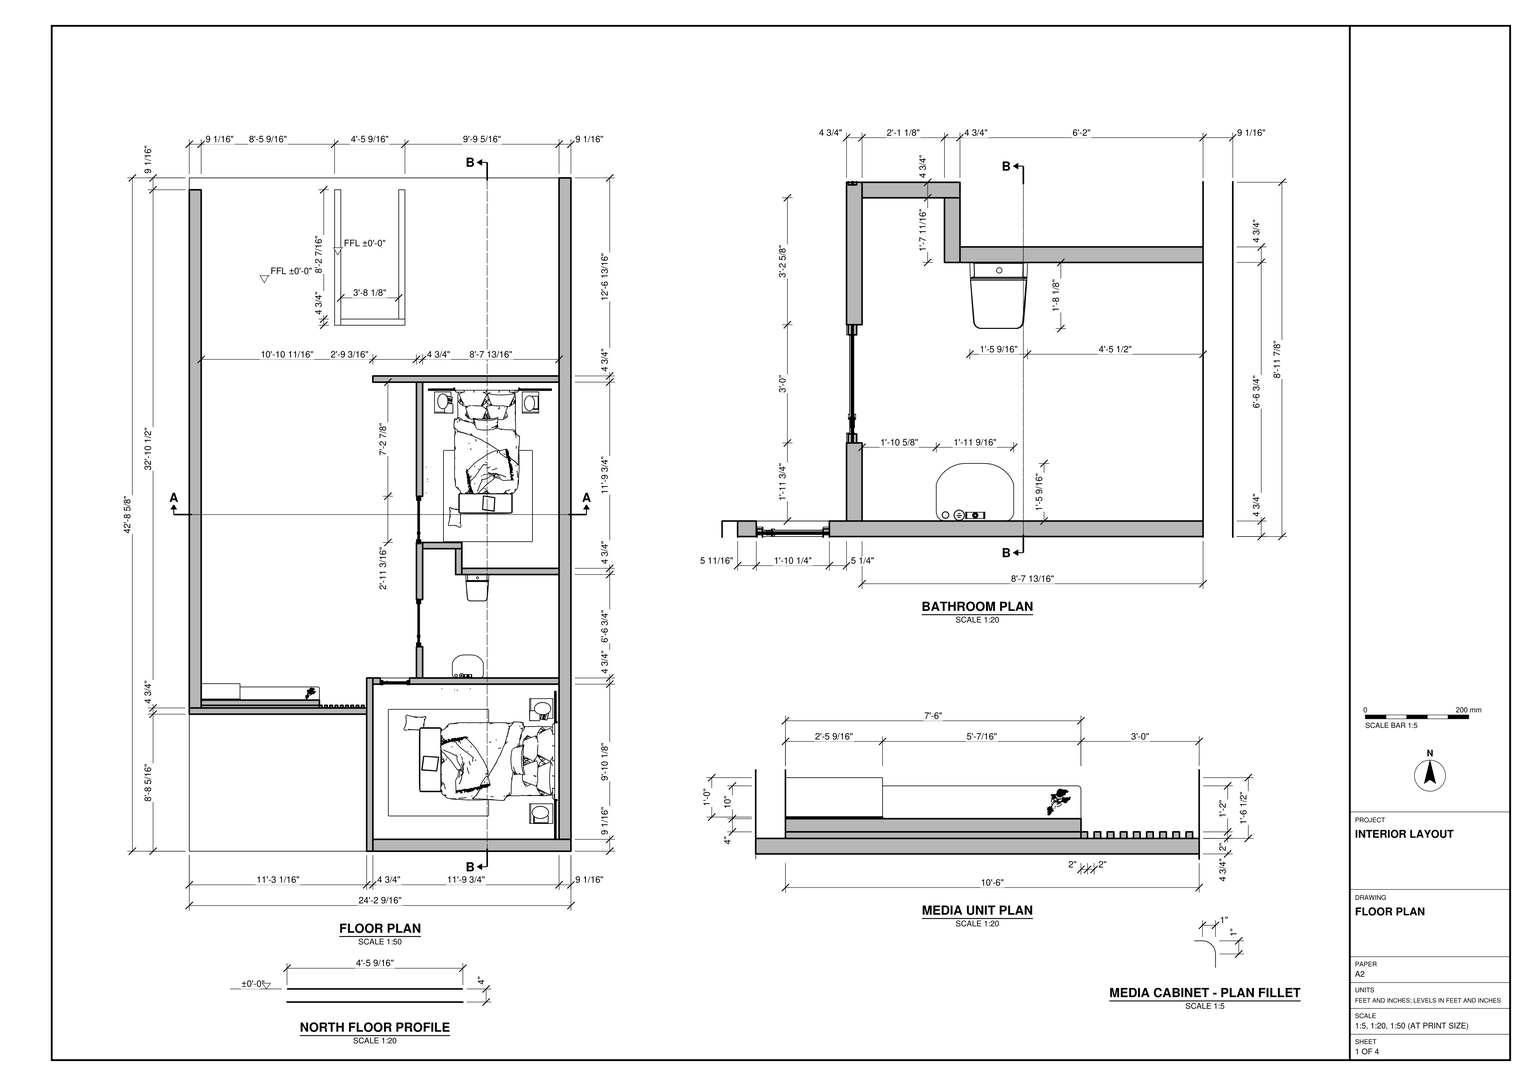
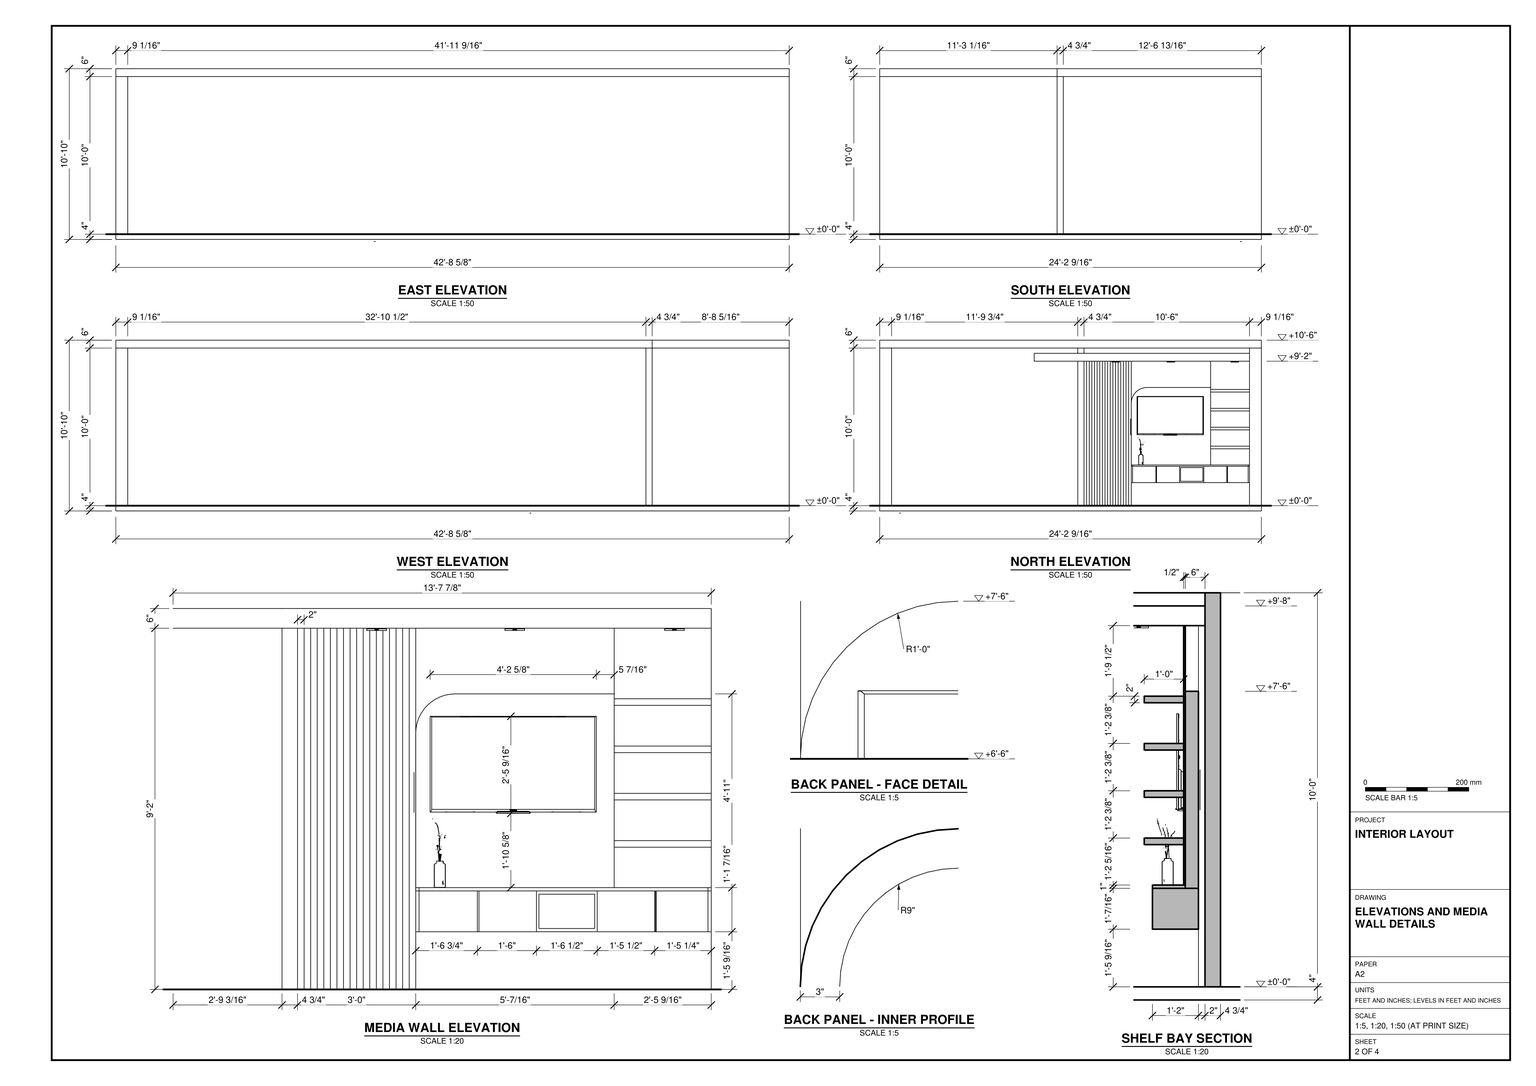
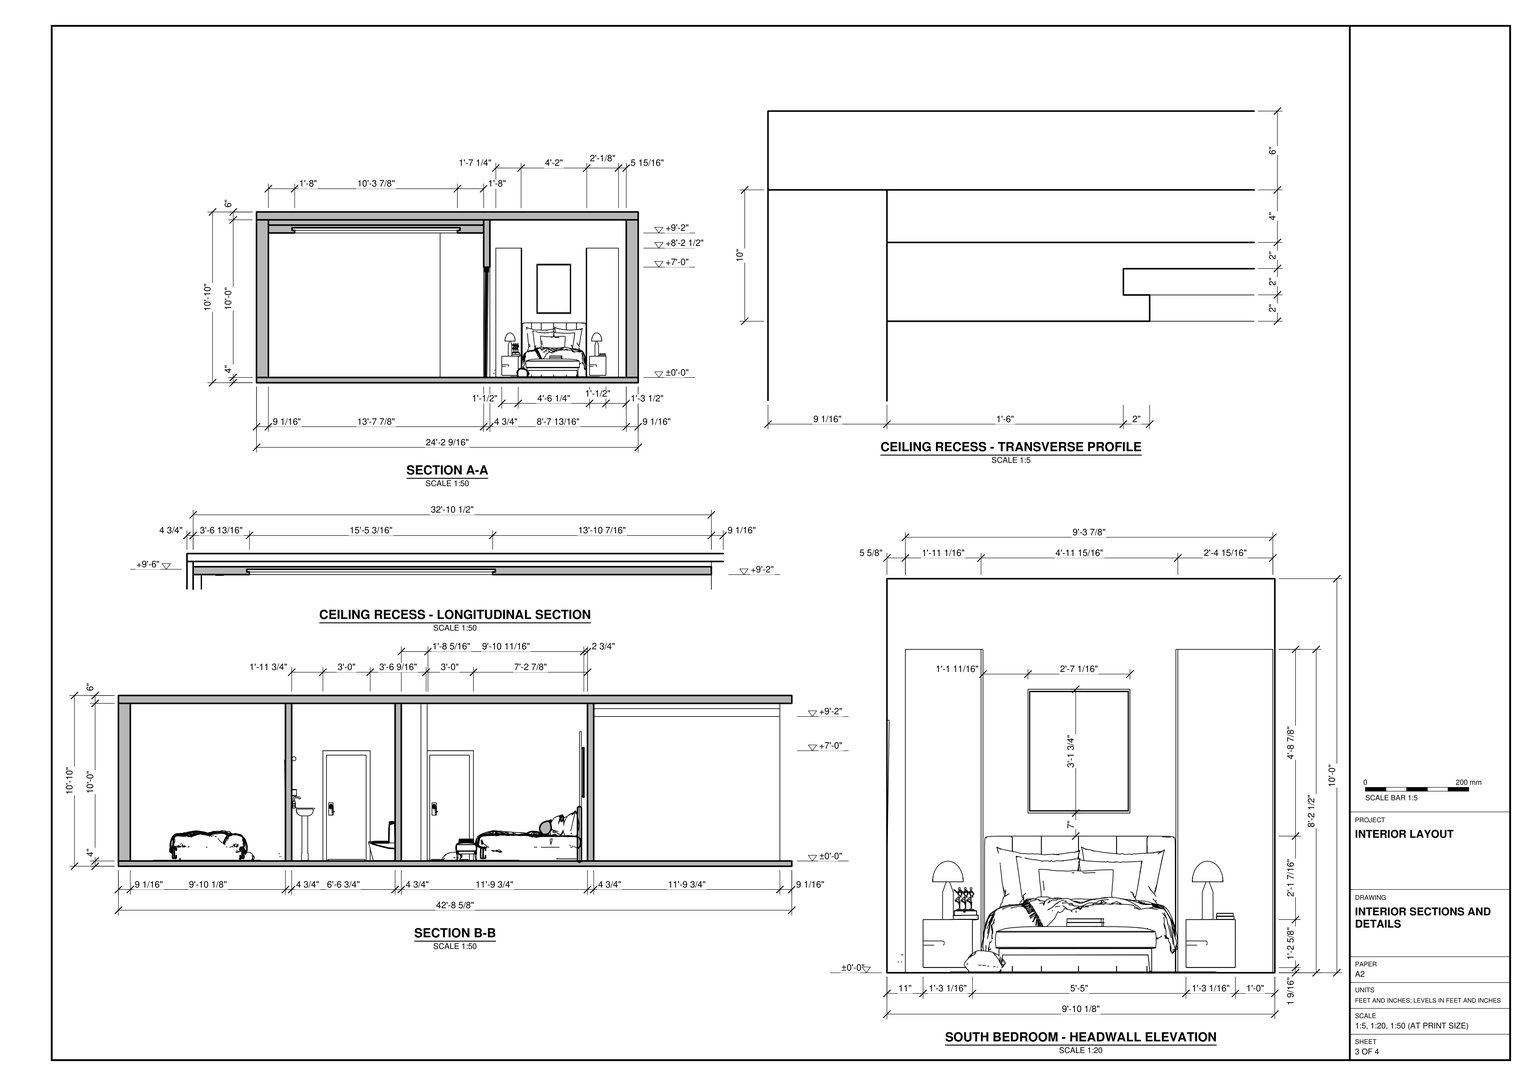
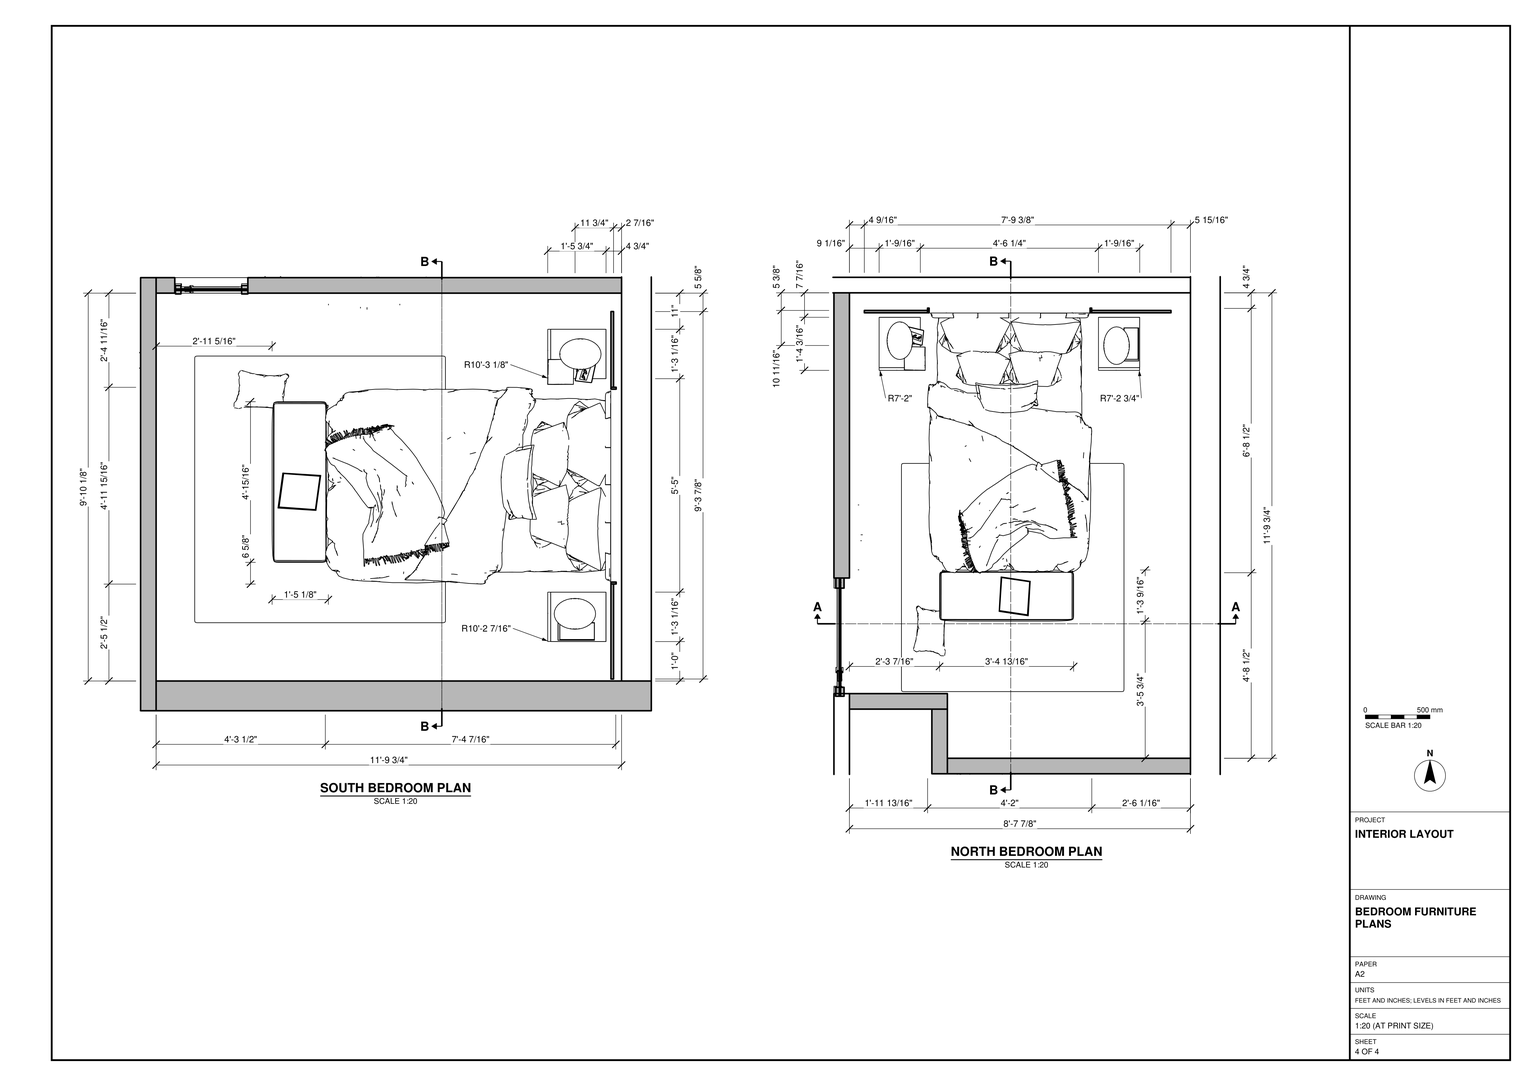
Build the furnished interior in SketchUp from task_files/diagram_01.pdf. Work in feet and inches. Set the finished floor at ±0'-0". The overall model is 24'-2 9/16" wide, 42'-8 5/8" long and 10'-10" high, including the floor and roof slabs.

Use the floor plan to set out the open area on the west and the two bedrooms on the east, with the bathroom between them. Follow the drawn wall thicknesses, partition returns and door openings, including the stepped wall behind the toilet. Match the north floor profile to the detail. Use the sections to establish the clear room height and to shape the stepped ceiling recess above the open area.

Place each bed and its bedside units in the orientation shown. Use the south bedroom elevation to size and position the headwall panels around the bed. Build the media wall from its plan, elevation and shelf section: distinguish the vertical slats, rounded screen back panel, suspended low cabinet and open shelf bay. Decor and loose items may be any suitable library components.

Keep the walls, slabs and roof as separate groups or components, and group each furniture or joinery piece separately. Use components for repeated parts. Save one SketchUp model as output_files/two_bedroom_interior_with_media_wall.skp.

# SketchUp Ruby script. Lengths in inches.
U = 1.inch
M = Sketchup.active_model
def pt(a) = Geom::Point3d.new(a.map { |v| v * U })
def face(e, loops, mat)
  f = e.add_face(loops[0].map { |a| pt(a) })
  loops[1..].each { |l| e.add_face(l.map { |a| pt(a) }).erase! }
  f.material = f.back_material = mat if mat
  f
end
# faces: each face lists its corners as indices into pts; further lists are holes
def faces(e, pts, list, mat = nil) = list.each { |f| face(e, (f[0].is_a?(Array) ? f : [f]).map { |l| l.map { |i| pts[i] } }, mat) }
# xy, xz, yz: faces in a plane at the given z, y or x. An outline is a flat list of corners, or four numbers for a rectangle; further outlines are holes
def ring(l) = l.size == 4 ? [[l[0], l[1]], [l[2], l[1]], [l[2], l[3]], [l[0], l[3]]] : l.each_slice(2).to_a
def flat(e, list, mat, &to3) = list.each { |f| face(e, (f[0].is_a?(Array) ? f : [f]).map { |l| ring(l).map { |u, v| to3.(u, v) } }, mat) }
def xy(e, z, list, mat = nil) = flat(e, list, mat) { |x, y| [x, y, z] }
def xz(e, y, list, mat = nil) = flat(e, list, mat) { |x, z| [x, y, z] }
def yz(e, x, list, mat = nil) = flat(e, list, mat) { |y, z| [x, y, z] }
def lines(e, pts, list) = list.each { |a, b| e.add_line(pt(pts[a]), pt(pts[b])) }
# prism: a flat outline (further loops are holes) pulled along v
def prism(e, loops, v, mat = nil)
  f = face(e, loops, mat); d = Geom::Vector3d.new(v.map { |x| x * U })
  f.pushpull(f.normal.samedirection?(d) ? d.length : -d.length)
end
def box(e, o, s, mat = nil) = prism(e, [[o, [o[0] + s[0], o[1], o[2]], [o[0] + s[0], o[1] + s[1], o[2]], [o[0], o[1] + s[1], o[2]]]], [0, 0, s[2]], mat)
def at(x, y, z, deg = 0) = Geom::Transformation.translation(pt([x, y, z])) * Geom::Transformation.rotation(ORIGIN, Z_AXIS, deg.degrees)
def axes(o, x, y, z) = Geom::Transformation.new([*x, 0, *y, 0, *z, 0, *pt(o).to_a, 1])
def part(name) = M.definitions.add(name)
# library, detail: a bought-in or finely detailed component or shape, given as its bounding box
def library(name, o, s) = part(name).tap { |d| box(d.entities, o, s) }
def detail(e, o, s) = box(e.add_group.entities, o, s)
def put(e, d, t, mat = nil) = e.add_instance(d, t).tap { |i| i.material = mat if mat }
def group(e, t, mat = nil) = e.add_group.tap { |g| g.transformation = t; g.material = mat if mat }.entities
root = M.entities
M.materials.add("0176 AP 7460 CRYSTAL RIVER").color = [209, 232, 226]
M.materials.add("0196 AP 8700 DIVINITY").color = [235, 221, 218]
M.materials.add("[Carrera Marble]").color = [207, 207, 207]
c1 = library("feets plan.dwg",[0,0,0],[290.55,512.6,0.01])
c2 = library("Nhatay-Combo+Bed-Modern+stylist+(35) (1)",[-205.01,128.15,-1.01],[153.05,130.41,99.44])
c3 = library("porta+4 (2)",[0.2,-5.42,1.33],[46.55,4.72,83.21])
c4 = library("3x5 small bath",[0,-13.07,0],[75.24,78.74,85])
c5 = part("Square post")
xy(c5.entities,0,[[0,0,2,2]])
xy(c5.entities,110,[[0,0,2,2]])
xz(c5.entities,0,[[0,0,2,110]])
xz(c5.entities,2,[[0,0,2,110]],"0176 AP 7460 CRYSTAL RIVER")
yz(c5.entities,0,[[0,0,2,110]],"0176 AP 7460 CRYSTAL RIVER")
yz(c5.entities,2,[[0,0,2,110]],"0176 AP 7460 CRYSTAL RIVER")
c6 = part("Shelf panel")
box(c6.entities,[0,0,0],[29.5625,12,2])
c7 = part("Group260\#1")
p = [[0,0,0],[0,0,-5.07],[-2.27,0,-5.07],[14.78,-1.625,0],[-14.78,-1.625,0],[14.78,1.625,0],
  [14.78,0,0],[-14.78,1.625,0],[2.27,0,-5.07],[-14.78,0,0],[0,0,-8.2]]
lines(c7.entities,p,[[0,1],[1,2],[3,4],[5,6],[7,5],[1,8],[9,0],[0,6],[8,10],[4,9],[6,3],[2,10],
  [9,7]])
c8 = part("Rectangle Light")
put(c8.entities,c7,at(0,0,0))
c9 = library("Flat panel television",[0,5.31,3.09],[110.25,6.46,64.42])
c10 = library("Sphere Light",[-21.15,-21.15,-21.15],[42.3,42.3,42.3])
c11 = library("Group\#21",[-0.5,-0.5,0],[91,4.5,60])
c12 = library("Group\#23",[-0.5,-0.5,-0.1],[128.88,190.2,0.2])
c13 = library("Group\#64",[-6.9375,-9.94,6.79],[29.29,38.38,46.85])
c14 = library("Group\#49",[0,0,0],[6,6,0.5])
put(root,c1,at(0,0,0))
put(root,c2,axes([23.37,-29.09,0.05],[0,-0.74598,0],[1,0,0],[0,0,1]))
put(root,c3,axes([145.56,131.89,0.12],[0.47368,0,0],[0,1,0],[0,0,0.90881]))
put(root,c4,at(275.5,197.5625,-5.625,-180))
put(root,c3,axes([171.1,155.51,-1.38],[0,0.77339,0],[-1,0,0],[0,0,1.01001]))
put(root,c3,axes([171.1,234.09,-1.38],[0,0.77339,0],[-1,0,0],[0,0,1.01001]))
put(root,c2,axes([307.9,119.04,0.05],[0.62245,0,0],[0,0.91,0],[0,0,1]))
put(root,c5,at(131.04,109.06,0))
put(root,c5,at(127.04,109.06,0))
put(root,c5,at(123.04,109.06,0))
put(root,c5,at(119.04,109.06,0))
put(root,c5,at(115.04,109.06,0))
put(root,c5,at(111.04,109.06,0))
put(root,c5,at(107.04,109.06,0))
put(root,c5,at(103.04,109.06,0))
put(root,c5,at(99.04,109.06,0))
put(root,c6,at(9.06,115.56,43.3125))
put(root,c6,at(9.06,115.56,57.71))
put(root,c6,at(9.06,115.56,72.11))
put(root,c6,at(9.06,115.56,86.51))
put(root,c8,at(23.84,117.18,86.5))
put(root,c8,at(23.84,117.18,72.1))
put(root,c8,at(23.84,117.18,57.7))
put(root,c8,at(23.84,117.18,43.3))
put(root,c9,axes([44.05,120.46,52.19],[0.45914,0,0],[0,-0.45914,0],[0,0,0.45914]))
put(root,c10,at(70.7,205.79,39.1875))
g1 = group(root,at(0,0,0))
xy(g1,-4,[[0,0,290.55,512.6]])
xy(g1,0,[[0,0,290.55,512.6]],"[Carrera Marble]")
xz(g1,0,[[0,-4,290.55,0]])
xz(g1,512.6,[[0,-4,290.55,0]])
yz(g1,0,[[0,-4,512.6,0]])
yz(g1,290.55,[[0,-4,512.6,0]])
g2 = group(root,at(281.5,9.06,0))
box(g2,[0,0,0],[9.06,503.54,120])
g3 = group(root,at(139.76,0,0))
box(g3,[0,0,0],[150.79,9.06,120])
g4 = group(root,at(135.04,0,0))
box(g4,[0,0,0],[4.72,131.89,120])
g5 = group(root,at(115.35,400.39,0))
xy(g5,0,[[0,0,48.82,4.72]])
g6 = group(root,at(110.63,400.39,0))
xy(g6,0,[[0,0,4.72,103.15]])
g7 = group(root,at(159.45,405.12,0))
xy(g7,0,[[0,0,4.72,98.43]])
g8 = group(root,at(139.76,357.09,0))
box(g8,[0,0,0],[141.73,4.72,120])
g9 = group(root,at(172.93,131.89,0))
prism(g9,[[[4.72,138.35,0],[4.72,225.2,0],[4.72,225.2,120],[4.72,0,120],[4.72,0,0],[4.72,23.78,0],[4.72,23.78,84],[4.72,59.78,84],[4.72,59.78,0],[4.72,103.15,0],[4.72,103.15,84],[4.72,138.35,84]]],[-4.72,0,0])
g10 = group(root,at(139.76,127.17,0))
xy(g10,0,[[0,0,5.6875,4.72],[5.6875,0,27.9375,4.72],[27.9375,0,141.73,4.72]])
xy(g10,76.95,[[5.6875,0,27.9375,4.72]])
xy(g10,120,[[0,0,141.73,4.72]])
xz(g10,0,[[0,0,5.6875,0,5.6875,76.95,27.9375,76.95,27.9375,0,141.73,0,141.73,120,0,120]])
xz(g10,4.72,[[0,0,0,120,141.73,120,141.73,0,27.9375,0,27.9375,76.95,5.6875,76.95,5.6875,0]])
yz(g10,0,[[0,0,4.72,120]])
yz(g10,5.6875,[[0,0,4.72,76.95]])
yz(g10,27.9375,[[0,0,4.72,76.95]])
yz(g10,141.73,[[0,0,4.72,120]])
g11 = group(root,at(0,104.33,0))
box(g11,[0,0,0],[135.04,4.72,120])
g12 = group(root,at(0,109.06,0))
box(g12,[0,0,0],[9.06,394.49,120])
g13 = group(root,at(207.48,210.63,0))
box(g13,[0,0,0],[74.02,4.72,120])
g14 = group(root,at(202.76,210.63,0))
box(g14,[0,0,0],[4.72,19.69,120])
g15 = group(root,at(177.66,230.31,0))
box(g15,[0,0,0],[29.82,4.72,120])
g16 = group(root,at(9.06,109.06,120))
prism(g16,[[[281.5,403.54,0],[281.5,-109.06,0],[125.98,-109.06,0],[125.98,-4.72,0],[-9.06,-4.72,0],[-9.06,403.54,0]]],[0,0,6])
put(root,c11,at(9.06,111.06,30))
g17 = group(root,at(9.06,109.06,112))
xy(g17,-2,[[[0,0,0,394.49,163.88,394.49,163.88,252.76,130.71,252.76,130.71,248.03,163.88,248.03,163.88,22.83,125.98,22.83,125.98,0],[20,42.83,143.88,228.03]]])
xy(g17,2,[[18,40.83,145.88,230.03]])
xy(g17,4,[[0,0,125.98,0,125.98,22.83,163.88,22.83,163.88,248.03,130.71,248.03,130.71,252.76,163.88,252.76,163.88,394.49,0,394.49]])
xz(g17,0,[[0,-2,125.98,4]])
xz(g17,22.83,[[125.98,-2,163.88,4]])
xz(g17,40.83,[[18,0,145.88,2]])
xz(g17,42.83,[[20,-2,143.88,0]])
xz(g17,228.03,[[20,-2,143.88,0]])
xz(g17,230.03,[[18,0,145.88,2]])
xz(g17,248.03,[[130.71,-2,163.88,4]])
xz(g17,252.76,[[130.71,-2,163.88,4]])
xz(g17,394.49,[[0,-2,163.88,4]])
yz(g17,0,[[0,-2,394.49,4]])
yz(g17,18,[[40.83,0,230.03,2]])
yz(g17,20,[[42.83,-2,228.03,0]])
yz(g17,125.98,[[0,-2,22.83,4]])
yz(g17,130.71,[[248.03,-2,252.76,4]])
yz(g17,143.88,[[42.83,-2,228.03,0]])
yz(g17,145.88,[[40.83,0,230.03,2]])
yz(g17,163.88,[[22.83,-2,248.03,4],[252.76,-2,394.49,4]])
put(g17,c12,at(18,40.83,0))
g18 = group(root,at(9.06,111.06,17.5625))
xy(g18,0,[[0,0,0,13,0.01,13.13,0.03,13.26,0.13,13.5,0.21,13.61,0.29,13.71,0.39,13.79,0.5,13.87,0.74,13.97,0.87,13.99,1,14,88.98,14,89.11,13.99,89.24,13.97,89.37,13.92,89.48,13.87,89.59,13.79,89.69,13.71,89.78,13.61,89.85,13.5,89.91,13.38,89.95,13.26,89.98,13.13,89.98,0]])
xy(g18,1,[[35.48,2,52.48,14]],"0176 AP 7460 CRYSTAL RIVER")
xy(g18,11.4375,[[35.48,2,52.48,14]],"0176 AP 7460 CRYSTAL RIVER")
xy(g18,12.4375,[[0,0,89.98,0,89.98,13.13,89.95,13.26,89.91,13.38,89.85,13.5,89.78,13.61,89.69,13.71,89.59,13.79,89.48,13.87,89.37,13.92,89.24,13.97,89.11,13.99,88.98,14,1,14,0.87,13.99,0.74,13.97,0.5,13.87,0.39,13.79,0.29,13.71,0.21,13.61,0.13,13.5,0.03,13.26,0.01,13.13,0,13]])
xz(g18,0,[[0,0,89.98,12.4375]])
xz(g18,2,[[35.48,1,52.48,11.4375]])
xz(g18,14,[[1,0,16.73,12.4375],[16.73,0,16.98,12.4375],[16.98,0,17.23,12.4375],[17.23,0,34.73,12.4375],[53.23,0,70.73,12.4375],
  [70.73,0,71.23,12.4375],[71.23,0,88.98,12.4375]])
xz(g18,14,[[[34.73,0,53.23,12.4375],[35.48,1,52.48,11.4375]]],"0176 AP 7460 CRYSTAL RIVER")
yz(g18,0,[[0,0,13,12.4375]])
yz(g18,35.48,[[2,1,14,11.4375]],"0176 AP 7460 CRYSTAL RIVER")
yz(g18,52.48,[[2,1,14,11.4375]],"0176 AP 7460 CRYSTAL RIVER")
yz(g18,89.98,[[0,0,13,12.4375],[13,0,13.13,12.4375]])
p = [[0,13,12.4375],[0.01,13.13,12.4375],[0.01,13.13,0],[0,13,0],[0.03,13.26,12.4375],[0.03,13.26,0],
  [89.95,13.26,12.4375],[89.98,13.13,12.4375],[89.98,13.13,0],[89.95,13.26,0],[0.08,13.38,12.4375],[0.08,13.38,0],
  [89.91,13.38,12.4375],[89.91,13.38,0],[0.13,13.5,12.4375],[0.13,13.5,0],[89.85,13.5,12.4375],[89.85,13.5,0],
  [0.21,13.61,12.4375],[0.21,13.61,0],[89.78,13.61,12.4375],[89.78,13.61,0],[0.29,13.71,12.4375],[0.29,13.71,0],
  [89.69,13.71,12.4375],[89.69,13.71,0],[0.39,13.79,12.4375],[0.39,13.79,0],[89.59,13.79,12.4375],[89.59,13.79,0],
  [0.5,13.87,12.4375],[0.5,13.87,0],[89.48,13.87,12.4375],[89.48,13.87,0],[0.62,13.92,12.4375],[0.62,13.92,0],
  [0.74,13.97,12.4375],[0.74,13.97,0],[89.24,13.97,12.4375],[89.37,13.92,12.4375],[89.37,13.92,0],[89.24,13.97,0],
  [0.87,13.99,12.4375],[0.87,13.99,0],[1,14,12.4375],[1,14,0],[88.98,14,12.4375],[89.11,13.99,12.4375],
  [89.11,13.99,0],[88.98,14,0]]
faces(g18,p,[[0,1,2,3],[1,4,5,2],[6,7,8,9],[4,10,11,5],[12,6,9,13],[10,14,15,11],[16,12,13,17],[14,18,19,15],
  [20,16,17,21],[18,22,23,19],[24,20,21,25],[22,26,27,23],[28,24,25,29],[26,30,31,27],[32,28,29,33],[30,34,35,31],
  [34,36,37,35],[38,39,40,41],[39,32,33,40],[36,42,43,37],[42,44,45,43],[46,47,48,49],[47,38,41,48]])
g19 = group(root,at(9.06,111.06,32),"0176 AP 7460 CRYSTAL RIVER")
prism(g19,[[[1,14,-2],[88.98,14,-2],[89.11,13.99,-2],[89.24,13.97,-2],[89.37,13.92,-2],[89.48,13.87,-2],[89.59,13.79,-2],[89.69,13.71,-2],[89.78,13.61,-2],[89.85,13.5,-2],[89.91,13.38,-2],[89.95,13.26,-2],[89.98,13.13,-2],[89.98,13,-2],[89.98,4,-2],[0,4,-2],[0,13,-2],[0.01,13.13,-2],[0.03,13.26,-2],[0.08,13.38,-2],[0.13,13.5,-2],[0.21,13.61,-2],[0.29,13.71,-2],[0.39,13.79,-2],[0.5,13.87,-2],[0.62,13.92,-2],[0.74,13.97,-2],[0.87,13.99,-2]]],[0,0,1])
g20 = group(root,at(9.06,115.06,31),"0196 AP 8700 DIVINITY")
box(g20,[0,0,0],[29.5625,0.5,79])
put(root,c13,axes([89.01,115.6,26.5],[-0.26315,0.45579,0],[0.45579,0.26315,0],[0,0,0.5263]))
put(root,c14,at(107.96,126.24,109.3125))
put(root,c14,at(65.89,126.24,109.3125))
put(root,c14,at(17.27,126.24,109.3125))
